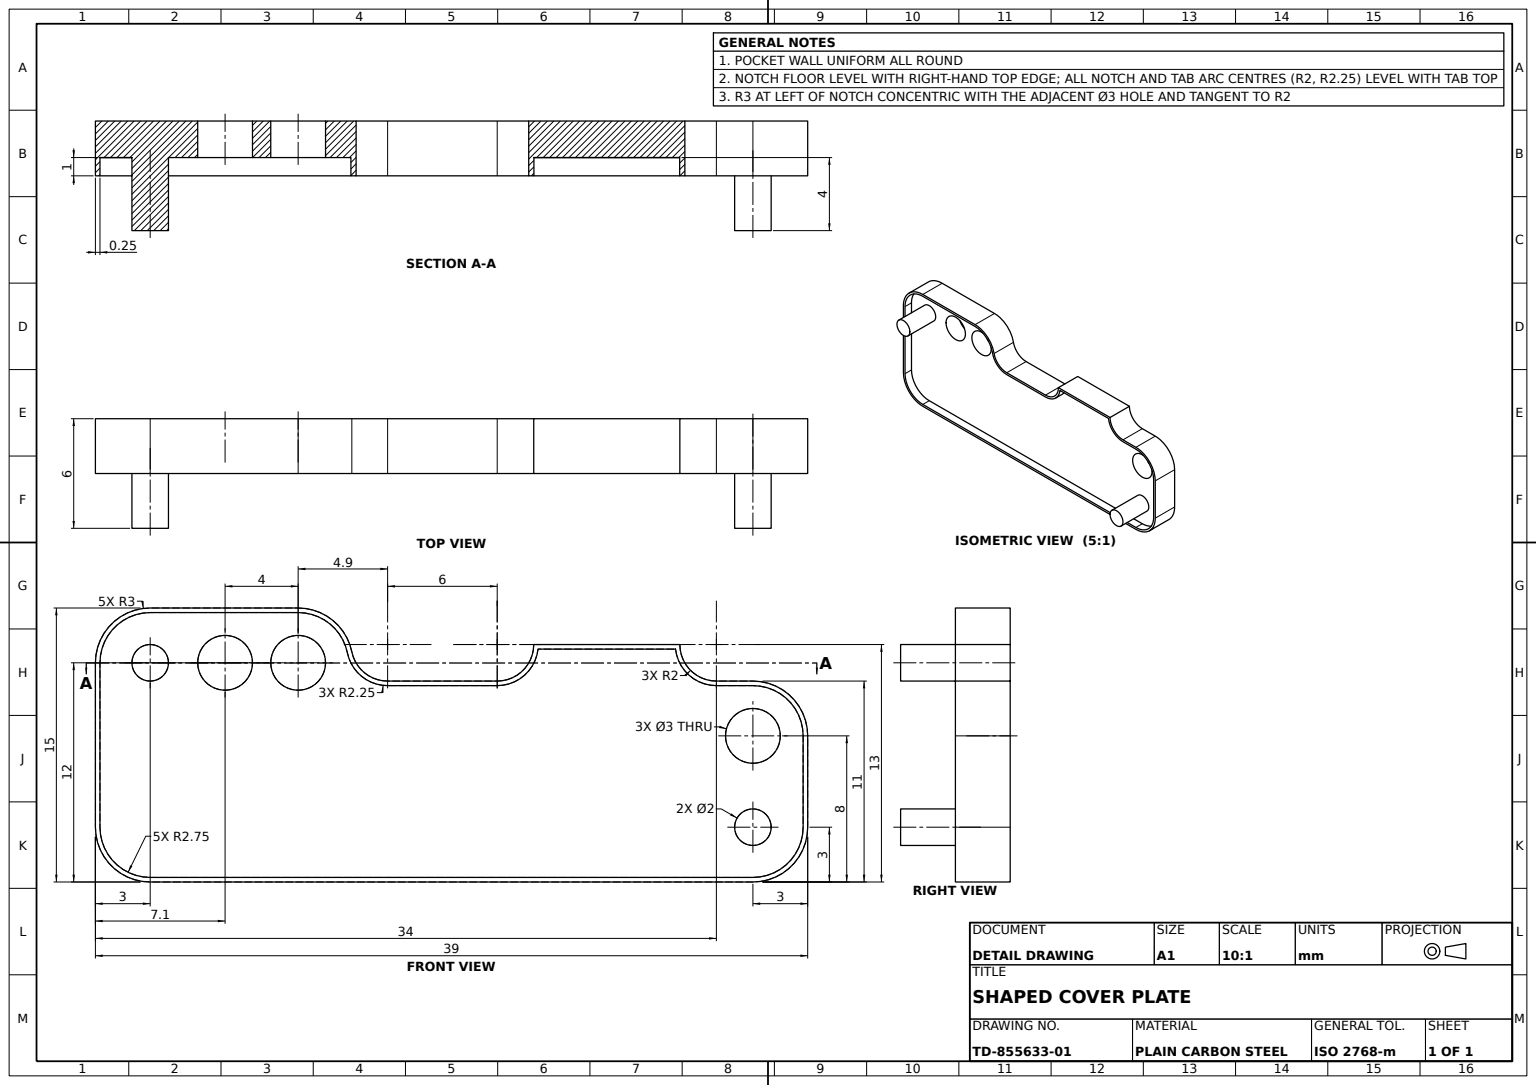
ISO-10303-21;
HEADER;
FILE_DESCRIPTION((''),'2;1');
FILE_NAME('','',(''),(''),'','','');
FILE_SCHEMA(('AUTOMOTIVE_DESIGN'));
ENDSEC;
DATA;
#1=APPLICATION_CONTEXT('');
#2=PRODUCT_CONTEXT('',#1,'mechanical');
#3=PRODUCT('','','',(#2));
#4=PRODUCT_DEFINITION_FORMATION('','',#3);
#5=PRODUCT_DEFINITION_CONTEXT('',#1,'design');
#6=PRODUCT_DEFINITION('','',#4,#5);
#7=PRODUCT_DEFINITION_SHAPE('','',#6);
#8=(LENGTH_UNIT()NAMED_UNIT(*)SI_UNIT(.MILLI.,.METRE.));
#9=(NAMED_UNIT(*)PLANE_ANGLE_UNIT()SI_UNIT($,.RADIAN.));
#10=(NAMED_UNIT(*)SI_UNIT($,.STERADIAN.)SOLID_ANGLE_UNIT());
#11=UNCERTAINTY_MEASURE_WITH_UNIT(LENGTH_MEASURE(1.E-05),#8,'distance_accuracy_value','');
#12=(GEOMETRIC_REPRESENTATION_CONTEXT(3)GLOBAL_UNCERTAINTY_ASSIGNED_CONTEXT((#11))GLOBAL_UNIT_ASSIGNED_CONTEXT((#8,#9,#10))REPRESENTATION_CONTEXT('',''));
#13=CARTESIAN_POINT('',(16.,10.75,2.));
#14=VERTEX_POINT('',#13);
#15=CARTESIAN_POINT('',(13.795459,12.55,2.));
#16=VERTEX_POINT('',#15);
#17=CARTESIAN_POINT('',(16.,13.,2.));
#18=DIRECTION('',(0.,0.,-1.));
#19=DIRECTION('',(1.,0.,0.));
#20=AXIS2_PLACEMENT_3D('',#17,#18,#19);
#21=CIRCLE('',#20,2.25);
#22=EDGE_CURVE('',#14,#16,#21,.T.);
#23=ORIENTED_EDGE('',*,*,#22,.F.);
#24=CARTESIAN_POINT('',(16.,10.75,3.));
#25=VERTEX_POINT('',#24);
#26=VECTOR('',#18,1000.);
#27=LINE('',#24,#26);
#28=EDGE_CURVE('',#25,#14,#27,.T.);
#29=ORIENTED_EDGE('',*,*,#28,.F.);
#30=CARTESIAN_POINT('',(13.795459,12.55,3.));
#31=VERTEX_POINT('',#30);
#32=CARTESIAN_POINT('',(16.,13.,3.));
#33=AXIS2_PLACEMENT_3D('',#32,#18,#19);
#34=CIRCLE('',#33,2.25);
#35=EDGE_CURVE('',#25,#31,#34,.T.);
#36=ORIENTED_EDGE('',*,*,#35,.T.);
#37=LINE('',#30,#26);
#38=EDGE_CURVE('',#31,#16,#37,.T.);
#39=ORIENTED_EDGE('',*,*,#38,.T.);
#40=EDGE_LOOP('',(#23,#29,#36,#39));
#41=FACE_OUTER_BOUND('',#40,.T.);
#42=DIRECTION('',(-1.,0.,0.));
#43=AXIS2_PLACEMENT_3D('',#32,#18,#42);
#44=CYLINDRICAL_SURFACE('',#43,2.25);
#45=ADVANCED_FACE('',(#41),#44,.T.);
#46=CARTESIAN_POINT('',(3.,15.,3.));
#47=VERTEX_POINT('',#46);
#48=CARTESIAN_POINT('',(3.,15.,0.));
#49=VERTEX_POINT('',#48);
#50=CARTESIAN_POINT('',(3.,15.,2.));
#51=LINE('',#50,#26);
#52=EDGE_CURVE('',#47,#49,#51,.T.);
#53=ORIENTED_EDGE('',*,*,#52,.F.);
#54=CARTESIAN_POINT('',(11.101021,15.,3.));
#55=VERTEX_POINT('',#54);
#56=VECTOR('',#42,1000.);
#57=LINE('',#54,#56);
#58=EDGE_CURVE('',#55,#47,#57,.T.);
#59=ORIENTED_EDGE('',*,*,#58,.F.);
#60=CARTESIAN_POINT('',(11.101021,15.,0.));
#61=VERTEX_POINT('',#60);
#62=CARTESIAN_POINT('',(11.101021,15.,2.));
#63=LINE('',#62,#26);
#64=EDGE_CURVE('',#55,#61,#63,.T.);
#65=ORIENTED_EDGE('',*,*,#64,.T.);
#66=LINE('',#60,#56);
#67=EDGE_CURVE('',#61,#49,#66,.T.);
#68=ORIENTED_EDGE('',*,*,#67,.T.);
#69=EDGE_LOOP('',(#53,#59,#65,#68));
#70=FACE_OUTER_BOUND('',#69,.T.);
#71=DIRECTION('',(0.,-1.,0.));
#72=AXIS2_PLACEMENT_3D('',#62,#71,#18);
#73=PLANE('',#72);
#74=ADVANCED_FACE('',(#70),#73,.F.);
#75=CARTESIAN_POINT('',(34.5,8.,0.));
#76=VERTEX_POINT('',#75);
#77=CARTESIAN_POINT('',(37.5,8.,0.));
#78=VERTEX_POINT('',#77);
#79=CARTESIAN_POINT('',(36.,8.,0.));
#80=DIRECTION('',(0.,0.,1.));
#81=AXIS2_PLACEMENT_3D('',#79,#80,#19);
#82=CIRCLE('',#81,1.5);
#83=EDGE_CURVE('',#76,#78,#82,.T.);
#84=ORIENTED_EDGE('',*,*,#83,.F.);
#85=CARTESIAN_POINT('',(34.5,8.,2.));
#86=VERTEX_POINT('',#85);
#87=CARTESIAN_POINT('',(34.5,8.,-2.));
#88=VECTOR('',#80,1000.);
#89=LINE('',#87,#88);
#90=EDGE_CURVE('',#76,#86,#89,.T.);
#91=ORIENTED_EDGE('',*,*,#90,.T.);
#92=CARTESIAN_POINT('',(37.5,8.,2.));
#93=VERTEX_POINT('',#92);
#94=CARTESIAN_POINT('',(36.,8.,2.));
#95=AXIS2_PLACEMENT_3D('',#94,#80,#19);
#96=CIRCLE('',#95,1.5);
#97=EDGE_CURVE('',#86,#93,#96,.T.);
#98=ORIENTED_EDGE('',*,*,#97,.T.);
#99=CARTESIAN_POINT('',(37.5,8.,-2.));
#100=LINE('',#99,#88);
#101=EDGE_CURVE('',#78,#93,#100,.T.);
#102=ORIENTED_EDGE('',*,*,#101,.F.);
#103=EDGE_LOOP('',(#84,#91,#98,#102));
#104=FACE_OUTER_BOUND('',#103,.T.);
#105=CARTESIAN_POINT('',(36.,8.,-2.));
#106=AXIS2_PLACEMENT_3D('',#105,#80,#19);
#107=CYLINDRICAL_SURFACE('',#106,1.5);
#108=ADVANCED_FACE('',(#104),#107,.F.);
#109=CARTESIAN_POINT('',(12.601021,12.,0.));
#110=VERTEX_POINT('',#109);
#111=CARTESIAN_POINT('',(9.601021,12.,0.));
#112=VERTEX_POINT('',#111);
#113=CARTESIAN_POINT('',(11.101021,12.,0.));
#114=AXIS2_PLACEMENT_3D('',#113,#80,#19);
#115=CIRCLE('',#114,1.5);
#116=EDGE_CURVE('',#110,#112,#115,.T.);
#117=ORIENTED_EDGE('',*,*,#116,.T.);
#118=EDGE_CURVE('',#112,#110,#115,.T.);
#119=ORIENTED_EDGE('',*,*,#118,.T.);
#120=EDGE_LOOP('',(#117,#119));
#121=FACE_BOUND('',#120,.T.);
#122=ORIENTED_EDGE('',*,*,#83,.T.);
#123=EDGE_CURVE('',#78,#76,#82,.T.);
#124=ORIENTED_EDGE('',*,*,#123,.T.);
#125=EDGE_LOOP('',(#122,#124));
#126=FACE_BOUND('',#125,.T.);
#127=CARTESIAN_POINT('',(5.601021,12.,0.));
#128=VERTEX_POINT('',#127);
#129=CARTESIAN_POINT('',(8.601021,12.,0.));
#130=VERTEX_POINT('',#129);
#131=CARTESIAN_POINT('',(7.101021,12.,0.));
#132=AXIS2_PLACEMENT_3D('',#131,#80,#19);
#133=CIRCLE('',#132,1.5);
#134=EDGE_CURVE('',#128,#130,#133,.T.);
#135=ORIENTED_EDGE('',*,*,#134,.T.);
#136=EDGE_CURVE('',#130,#128,#133,.T.);
#137=ORIENTED_EDGE('',*,*,#136,.T.);
#138=EDGE_LOOP('',(#135,#137));
#139=FACE_BOUND('',#138,.T.);
#140=CARTESIAN_POINT('',(0.,12.,0.));
#141=VERTEX_POINT('',#140);
#142=CARTESIAN_POINT('',(0.,3.,0.));
#143=VERTEX_POINT('',#142);
#144=VECTOR('',#71,1000.);
#145=LINE('',#142,#144);
#146=EDGE_CURVE('',#141,#143,#145,.T.);
#147=ORIENTED_EDGE('',*,*,#146,.F.);
#148=CARTESIAN_POINT('',(3.,12.,0.));
#149=AXIS2_PLACEMENT_3D('',#148,#80,#42);
#150=CIRCLE('',#149,3.);
#151=EDGE_CURVE('',#49,#141,#150,.T.);
#152=ORIENTED_EDGE('',*,*,#151,.F.);
#153=ORIENTED_EDGE('',*,*,#67,.F.);
#154=CARTESIAN_POINT('',(14.040408,12.6,0.));
#155=VERTEX_POINT('',#154);
#156=CIRCLE('',#114,3.);
#157=EDGE_CURVE('',#155,#61,#156,.T.);
#158=ORIENTED_EDGE('',*,*,#157,.F.);
#159=CARTESIAN_POINT('',(16.,11.,0.));
#160=VERTEX_POINT('',#159);
#161=CARTESIAN_POINT('',(16.,13.,0.));
#162=AXIS2_PLACEMENT_3D('',#161,#18,#42);
#163=CIRCLE('',#162,2.);
#164=EDGE_CURVE('',#160,#155,#163,.T.);
#165=ORIENTED_EDGE('',*,*,#164,.F.);
#166=CARTESIAN_POINT('',(22.,11.,0.));
#167=VERTEX_POINT('',#166);
#168=LINE('',#166,#56);
#169=EDGE_CURVE('',#167,#160,#168,.T.);
#170=ORIENTED_EDGE('',*,*,#169,.F.);
#171=CARTESIAN_POINT('',(24.,13.,0.));
#172=VERTEX_POINT('',#171);
#173=CARTESIAN_POINT('',(22.,13.,0.));
#174=AXIS2_PLACEMENT_3D('',#173,#18,#19);
#175=CIRCLE('',#174,2.);
#176=EDGE_CURVE('',#172,#167,#175,.T.);
#177=ORIENTED_EDGE('',*,*,#176,.F.);
#178=CARTESIAN_POINT('',(32.,13.,0.));
#179=VERTEX_POINT('',#178);
#180=LINE('',#178,#56);
#181=EDGE_CURVE('',#179,#172,#180,.T.);
#182=ORIENTED_EDGE('',*,*,#181,.F.);
#183=CARTESIAN_POINT('',(34.,11.,0.));
#184=VERTEX_POINT('',#183);
#185=CARTESIAN_POINT('',(34.,13.,0.));
#186=AXIS2_PLACEMENT_3D('',#185,#18,#19);
#187=CIRCLE('',#186,2.);
#188=EDGE_CURVE('',#184,#179,#187,.T.);
#189=ORIENTED_EDGE('',*,*,#188,.F.);
#190=CARTESIAN_POINT('',(36.,11.,0.));
#191=VERTEX_POINT('',#190);
#192=LINE('',#190,#56);
#193=EDGE_CURVE('',#191,#184,#192,.T.);
#194=ORIENTED_EDGE('',*,*,#193,.F.);
#195=CARTESIAN_POINT('',(39.,8.,0.));
#196=VERTEX_POINT('',#195);
#197=CIRCLE('',#81,3.);
#198=EDGE_CURVE('',#196,#191,#197,.T.);
#199=ORIENTED_EDGE('',*,*,#198,.F.);
#200=CARTESIAN_POINT('',(39.,3.,0.));
#201=VERTEX_POINT('',#200);
#202=DIRECTION('',(0.,1.,0.));
#203=VECTOR('',#202,1000.);
#204=LINE('',#200,#203);
#205=EDGE_CURVE('',#201,#196,#204,.T.);
#206=ORIENTED_EDGE('',*,*,#205,.F.);
#207=CARTESIAN_POINT('',(36.,0.,0.));
#208=VERTEX_POINT('',#207);
#209=CARTESIAN_POINT('',(36.,3.,0.));
#210=AXIS2_PLACEMENT_3D('',#209,#80,#19);
#211=CIRCLE('',#210,3.);
#212=EDGE_CURVE('',#208,#201,#211,.T.);
#213=ORIENTED_EDGE('',*,*,#212,.F.);
#214=CARTESIAN_POINT('',(3.,0.,0.));
#215=VERTEX_POINT('',#214);
#216=VECTOR('',#19,1000.);
#217=LINE('',#214,#216);
#218=EDGE_CURVE('',#215,#208,#217,.T.);
#219=ORIENTED_EDGE('',*,*,#218,.F.);
#220=CARTESIAN_POINT('',(3.,3.,0.));
#221=AXIS2_PLACEMENT_3D('',#220,#80,#19);
#222=CIRCLE('',#221,3.);
#223=EDGE_CURVE('',#143,#215,#222,.T.);
#224=ORIENTED_EDGE('',*,*,#223,.F.);
#225=EDGE_LOOP('',(#147,#152,#153,#158,#165,#170,#177,#182,#189,#194,#199,#206,#213,#219,#224));
#226=FACE_OUTER_BOUND('',#225,.T.);
#227=AXIS2_PLACEMENT_3D('',#185,#80,#19);
#228=PLANE('',#227);
#229=ADVANCED_FACE('',(#121,#126,#139,#226),#228,.F.);
#230=CARTESIAN_POINT('',(3.,14.75,3.));
#231=VERTEX_POINT('',#230);
#232=CARTESIAN_POINT('',(0.25,12.,3.));
#233=VERTEX_POINT('',#232);
#234=CARTESIAN_POINT('',(3.,12.,3.));
#235=AXIS2_PLACEMENT_3D('',#234,#80,#19);
#236=CIRCLE('',#235,2.75);
#237=EDGE_CURVE('',#231,#233,#236,.T.);
#238=ORIENTED_EDGE('',*,*,#237,.T.);
#239=CARTESIAN_POINT('',(0.25,12.,2.));
#240=VERTEX_POINT('',#239);
#241=LINE('',#232,#26);
#242=EDGE_CURVE('',#233,#240,#241,.T.);
#243=ORIENTED_EDGE('',*,*,#242,.T.);
#244=CARTESIAN_POINT('',(3.,14.75,2.));
#245=VERTEX_POINT('',#244);
#246=CARTESIAN_POINT('',(3.,12.,2.));
#247=AXIS2_PLACEMENT_3D('',#246,#80,#19);
#248=CIRCLE('',#247,2.75);
#249=EDGE_CURVE('',#245,#240,#248,.T.);
#250=ORIENTED_EDGE('',*,*,#249,.F.);
#251=LINE('',#230,#26);
#252=EDGE_CURVE('',#231,#245,#251,.T.);
#253=ORIENTED_EDGE('',*,*,#252,.F.);
#254=EDGE_LOOP('',(#238,#243,#250,#253));
#255=FACE_OUTER_BOUND('',#254,.T.);
#256=AXIS2_PLACEMENT_3D('',#234,#18,#42);
#257=CYLINDRICAL_SURFACE('',#256,2.75);
#258=ADVANCED_FACE('',(#255),#257,.F.);
#259=CARTESIAN_POINT('',(0.25,3.,3.));
#260=VERTEX_POINT('',#259);
#261=CARTESIAN_POINT('',(0.25,3.,2.));
#262=VERTEX_POINT('',#261);
#263=LINE('',#259,#26);
#264=EDGE_CURVE('',#260,#262,#263,.T.);
#265=ORIENTED_EDGE('',*,*,#264,.F.);
#266=CARTESIAN_POINT('',(3.,0.25,3.));
#267=VERTEX_POINT('',#266);
#268=CARTESIAN_POINT('',(3.,3.,3.));
#269=AXIS2_PLACEMENT_3D('',#268,#80,#19);
#270=CIRCLE('',#269,2.75);
#271=EDGE_CURVE('',#260,#267,#270,.T.);
#272=ORIENTED_EDGE('',*,*,#271,.T.);
#273=CARTESIAN_POINT('',(3.,0.25,2.));
#274=VERTEX_POINT('',#273);
#275=LINE('',#266,#26);
#276=EDGE_CURVE('',#267,#274,#275,.T.);
#277=ORIENTED_EDGE('',*,*,#276,.T.);
#278=CARTESIAN_POINT('',(3.,3.,2.));
#279=AXIS2_PLACEMENT_3D('',#278,#80,#19);
#280=CIRCLE('',#279,2.75);
#281=EDGE_CURVE('',#262,#274,#280,.T.);
#282=ORIENTED_EDGE('',*,*,#281,.F.);
#283=EDGE_LOOP('',(#265,#272,#277,#282));
#284=FACE_OUTER_BOUND('',#283,.T.);
#285=AXIS2_PLACEMENT_3D('',#268,#18,#42);
#286=CYLINDRICAL_SURFACE('',#285,2.75);
#287=ADVANCED_FACE('',(#284),#286,.F.);
#288=ORIENTED_EDGE('',*,*,#58,.T.);
#289=CARTESIAN_POINT('',(0.,12.,3.));
#290=VERTEX_POINT('',#289);
#291=CIRCLE('',#235,3.);
#292=EDGE_CURVE('',#47,#290,#291,.T.);
#293=ORIENTED_EDGE('',*,*,#292,.T.);
#294=CARTESIAN_POINT('',(0.,3.,3.));
#295=VERTEX_POINT('',#294);
#296=LINE('',#289,#144);
#297=EDGE_CURVE('',#290,#295,#296,.T.);
#298=ORIENTED_EDGE('',*,*,#297,.T.);
#299=CARTESIAN_POINT('',(3.,0.,3.));
#300=VERTEX_POINT('',#299);
#301=CIRCLE('',#269,3.);
#302=EDGE_CURVE('',#295,#300,#301,.T.);
#303=ORIENTED_EDGE('',*,*,#302,.T.);
#304=CARTESIAN_POINT('',(36.,0.,3.));
#305=VERTEX_POINT('',#304);
#306=LINE('',#299,#216);
#307=EDGE_CURVE('',#300,#305,#306,.T.);
#308=ORIENTED_EDGE('',*,*,#307,.T.);
#309=CARTESIAN_POINT('',(39.,3.,3.));
#310=VERTEX_POINT('',#309);
#311=CARTESIAN_POINT('',(36.,3.,3.));
#312=AXIS2_PLACEMENT_3D('',#311,#80,#19);
#313=CIRCLE('',#312,3.);
#314=EDGE_CURVE('',#305,#310,#313,.T.);
#315=ORIENTED_EDGE('',*,*,#314,.T.);
#316=CARTESIAN_POINT('',(39.,8.,3.));
#317=VERTEX_POINT('',#316);
#318=LINE('',#309,#203);
#319=EDGE_CURVE('',#310,#317,#318,.T.);
#320=ORIENTED_EDGE('',*,*,#319,.T.);
#321=CARTESIAN_POINT('',(36.,11.,3.));
#322=VERTEX_POINT('',#321);
#323=CARTESIAN_POINT('',(36.,8.,3.));
#324=AXIS2_PLACEMENT_3D('',#323,#80,#19);
#325=CIRCLE('',#324,3.);
#326=EDGE_CURVE('',#317,#322,#325,.T.);
#327=ORIENTED_EDGE('',*,*,#326,.T.);
#328=CARTESIAN_POINT('',(34.,11.,3.));
#329=VERTEX_POINT('',#328);
#330=LINE('',#321,#56);
#331=EDGE_CURVE('',#322,#329,#330,.T.);
#332=ORIENTED_EDGE('',*,*,#331,.T.);
#333=CARTESIAN_POINT('',(32.,13.,3.));
#334=VERTEX_POINT('',#333);
#335=CARTESIAN_POINT('',(34.,13.,3.));
#336=AXIS2_PLACEMENT_3D('',#335,#18,#19);
#337=CIRCLE('',#336,2.);
#338=EDGE_CURVE('',#329,#334,#337,.T.);
#339=ORIENTED_EDGE('',*,*,#338,.T.);
#340=CARTESIAN_POINT('',(24.,13.,3.));
#341=VERTEX_POINT('',#340);
#342=LINE('',#333,#56);
#343=EDGE_CURVE('',#334,#341,#342,.T.);
#344=ORIENTED_EDGE('',*,*,#343,.T.);
#345=CARTESIAN_POINT('',(22.,11.,3.));
#346=VERTEX_POINT('',#345);
#347=CARTESIAN_POINT('',(22.,13.,3.));
#348=AXIS2_PLACEMENT_3D('',#347,#18,#19);
#349=CIRCLE('',#348,2.);
#350=EDGE_CURVE('',#341,#346,#349,.T.);
#351=ORIENTED_EDGE('',*,*,#350,.T.);
#352=CARTESIAN_POINT('',(16.,11.,3.));
#353=VERTEX_POINT('',#352);
#354=LINE('',#345,#56);
#355=EDGE_CURVE('',#346,#353,#354,.T.);
#356=ORIENTED_EDGE('',*,*,#355,.T.);
#357=CARTESIAN_POINT('',(14.040408,12.6,3.));
#358=VERTEX_POINT('',#357);
#359=CIRCLE('',#33,2.);
#360=EDGE_CURVE('',#353,#358,#359,.T.);
#361=ORIENTED_EDGE('',*,*,#360,.T.);
#362=CARTESIAN_POINT('',(11.101021,12.,3.));
#363=AXIS2_PLACEMENT_3D('',#362,#80,#19);
#364=CIRCLE('',#363,3.);
#365=EDGE_CURVE('',#358,#55,#364,.T.);
#366=ORIENTED_EDGE('',*,*,#365,.T.);
#367=EDGE_LOOP('',(#288,#293,#298,#303,#308,#315,#320,#327,#332,#339,#344,#351,#356,#361,#366));
#368=FACE_OUTER_BOUND('',#367,.T.);
#369=CARTESIAN_POINT('',(38.75,8.,3.));
#370=VERTEX_POINT('',#369);
#371=CARTESIAN_POINT('',(36.,10.75,3.));
#372=VERTEX_POINT('',#371);
#373=CIRCLE('',#324,2.75);
#374=EDGE_CURVE('',#370,#372,#373,.T.);
#375=ORIENTED_EDGE('',*,*,#374,.F.);
#376=CARTESIAN_POINT('',(38.75,3.,3.));
#377=VERTEX_POINT('',#376);
#378=LINE('',#376,#203);
#379=EDGE_CURVE('',#377,#370,#378,.T.);
#380=ORIENTED_EDGE('',*,*,#379,.F.);
#381=CARTESIAN_POINT('',(36.,0.25,3.));
#382=VERTEX_POINT('',#381);
#383=CIRCLE('',#312,2.75);
#384=EDGE_CURVE('',#382,#377,#383,.T.);
#385=ORIENTED_EDGE('',*,*,#384,.F.);
#386=LINE('',#266,#216);
#387=EDGE_CURVE('',#267,#382,#386,.T.);
#388=ORIENTED_EDGE('',*,*,#387,.F.);
#389=ORIENTED_EDGE('',*,*,#271,.F.);
#390=LINE('',#232,#144);
#391=EDGE_CURVE('',#233,#260,#390,.T.);
#392=ORIENTED_EDGE('',*,*,#391,.F.);
#393=ORIENTED_EDGE('',*,*,#237,.F.);
#394=CARTESIAN_POINT('',(11.101021,14.75,3.));
#395=VERTEX_POINT('',#394);
#396=LINE('',#394,#56);
#397=EDGE_CURVE('',#395,#231,#396,.T.);
#398=ORIENTED_EDGE('',*,*,#397,.F.);
#399=CIRCLE('',#363,2.75);
#400=EDGE_CURVE('',#31,#395,#399,.T.);
#401=ORIENTED_EDGE('',*,*,#400,.F.);
#402=ORIENTED_EDGE('',*,*,#35,.F.);
#403=CARTESIAN_POINT('',(22.,10.75,3.));
#404=VERTEX_POINT('',#403);
#405=LINE('',#403,#56);
#406=EDGE_CURVE('',#404,#25,#405,.T.);
#407=ORIENTED_EDGE('',*,*,#406,.F.);
#408=CARTESIAN_POINT('',(24.236068,12.75,3.));
#409=VERTEX_POINT('',#408);
#410=CIRCLE('',#348,2.25);
#411=EDGE_CURVE('',#409,#404,#410,.T.);
#412=ORIENTED_EDGE('',*,*,#411,.F.);
#413=CARTESIAN_POINT('',(31.763932,12.75,3.));
#414=VERTEX_POINT('',#413);
#415=LINE('',#413,#56);
#416=EDGE_CURVE('',#414,#409,#415,.T.);
#417=ORIENTED_EDGE('',*,*,#416,.F.);
#418=CARTESIAN_POINT('',(34.,10.75,3.));
#419=VERTEX_POINT('',#418);
#420=CIRCLE('',#336,2.25);
#421=EDGE_CURVE('',#419,#414,#420,.T.);
#422=ORIENTED_EDGE('',*,*,#421,.F.);
#423=LINE('',#371,#56);
#424=EDGE_CURVE('',#372,#419,#423,.T.);
#425=ORIENTED_EDGE('',*,*,#424,.F.);
#426=EDGE_LOOP('',(#375,#380,#385,#388,#389,#392,#393,#398,#401,#402,#407,#412,#417,#422,#425));
#427=FACE_BOUND('',#426,.T.);
#428=AXIS2_PLACEMENT_3D('',#335,#80,#19);
#429=PLANE('',#428);
#430=ADVANCED_FACE('',(#368,#427),#429,.T.);
#431=ORIENTED_EDGE('',*,*,#400,.T.);
#432=CARTESIAN_POINT('',(11.101021,14.75,2.));
#433=VERTEX_POINT('',#432);
#434=LINE('',#394,#26);
#435=EDGE_CURVE('',#395,#433,#434,.T.);
#436=ORIENTED_EDGE('',*,*,#435,.T.);
#437=CARTESIAN_POINT('',(11.101021,12.,2.));
#438=AXIS2_PLACEMENT_3D('',#437,#80,#19);
#439=CIRCLE('',#438,2.75);
#440=EDGE_CURVE('',#16,#433,#439,.T.);
#441=ORIENTED_EDGE('',*,*,#440,.F.);
#442=ORIENTED_EDGE('',*,*,#38,.F.);
#443=EDGE_LOOP('',(#431,#436,#441,#442));
#444=FACE_OUTER_BOUND('',#443,.T.);
#445=AXIS2_PLACEMENT_3D('',#362,#18,#42);
#446=CYLINDRICAL_SURFACE('',#445,2.75);
#447=ADVANCED_FACE('',(#444),#446,.F.);
#448=CARTESIAN_POINT('',(34.,10.75,2.));
#449=VERTEX_POINT('',#448);
#450=LINE('',#418,#26);
#451=EDGE_CURVE('',#419,#449,#450,.T.);
#452=ORIENTED_EDGE('',*,*,#451,.F.);
#453=ORIENTED_EDGE('',*,*,#421,.T.);
#454=CARTESIAN_POINT('',(31.763932,12.75,2.));
#455=VERTEX_POINT('',#454);
#456=LINE('',#413,#26);
#457=EDGE_CURVE('',#414,#455,#456,.T.);
#458=ORIENTED_EDGE('',*,*,#457,.T.);
#459=CARTESIAN_POINT('',(34.,13.,2.));
#460=AXIS2_PLACEMENT_3D('',#459,#18,#19);
#461=CIRCLE('',#460,2.25);
#462=EDGE_CURVE('',#449,#455,#461,.T.);
#463=ORIENTED_EDGE('',*,*,#462,.F.);
#464=EDGE_LOOP('',(#452,#453,#458,#463));
#465=FACE_OUTER_BOUND('',#464,.T.);
#466=AXIS2_PLACEMENT_3D('',#335,#18,#42);
#467=CYLINDRICAL_SURFACE('',#466,2.25);
#468=ADVANCED_FACE('',(#465),#467,.T.);
#469=CARTESIAN_POINT('',(12.601021,12.,2.));
#470=VERTEX_POINT('',#469);
#471=CARTESIAN_POINT('',(12.601021,12.,-2.));
#472=LINE('',#471,#88);
#473=EDGE_CURVE('',#110,#470,#472,.T.);
#474=ORIENTED_EDGE('',*,*,#473,.F.);
#475=ORIENTED_EDGE('',*,*,#118,.F.);
#476=CARTESIAN_POINT('',(9.601021,12.,2.));
#477=VERTEX_POINT('',#476);
#478=CARTESIAN_POINT('',(9.601021,12.,-2.));
#479=LINE('',#478,#88);
#480=EDGE_CURVE('',#112,#477,#479,.T.);
#481=ORIENTED_EDGE('',*,*,#480,.T.);
#482=CIRCLE('',#438,1.5);
#483=EDGE_CURVE('',#477,#470,#482,.T.);
#484=ORIENTED_EDGE('',*,*,#483,.T.);
#485=EDGE_LOOP('',(#474,#475,#481,#484));
#486=FACE_OUTER_BOUND('',#485,.T.);
#487=CARTESIAN_POINT('',(11.101021,12.,-2.));
#488=AXIS2_PLACEMENT_3D('',#487,#80,#19);
#489=CYLINDRICAL_SURFACE('',#488,1.5);
#490=ADVANCED_FACE('',(#486),#489,.F.);
#491=CARTESIAN_POINT('',(16.,11.,2.));
#492=LINE('',#491,#26);
#493=EDGE_CURVE('',#353,#160,#492,.T.);
#494=ORIENTED_EDGE('',*,*,#493,.T.);
#495=ORIENTED_EDGE('',*,*,#164,.T.);
#496=CARTESIAN_POINT('',(14.040408,12.6,2.));
#497=LINE('',#496,#26);
#498=EDGE_CURVE('',#358,#155,#497,.T.);
#499=ORIENTED_EDGE('',*,*,#498,.F.);
#500=ORIENTED_EDGE('',*,*,#360,.F.);
#501=EDGE_LOOP('',(#494,#495,#499,#500));
#502=FACE_OUTER_BOUND('',#501,.T.);
#503=AXIS2_PLACEMENT_3D('',#17,#18,#42);
#504=CYLINDRICAL_SURFACE('',#503,2.);
#505=ADVANCED_FACE('',(#502),#504,.F.);
#506=ORIENTED_EDGE('',*,*,#374,.T.);
#507=CARTESIAN_POINT('',(36.,10.75,2.));
#508=VERTEX_POINT('',#507);
#509=LINE('',#371,#26);
#510=EDGE_CURVE('',#372,#508,#509,.T.);
#511=ORIENTED_EDGE('',*,*,#510,.T.);
#512=CARTESIAN_POINT('',(38.75,8.,2.));
#513=VERTEX_POINT('',#512);
#514=CIRCLE('',#95,2.75);
#515=EDGE_CURVE('',#513,#508,#514,.T.);
#516=ORIENTED_EDGE('',*,*,#515,.F.);
#517=LINE('',#369,#26);
#518=EDGE_CURVE('',#370,#513,#517,.T.);
#519=ORIENTED_EDGE('',*,*,#518,.F.);
#520=EDGE_LOOP('',(#506,#511,#516,#519));
#521=FACE_OUTER_BOUND('',#520,.T.);
#522=AXIS2_PLACEMENT_3D('',#323,#18,#42);
#523=CYLINDRICAL_SURFACE('',#522,2.75);
#524=ADVANCED_FACE('',(#521),#523,.F.);
#525=ORIENTED_EDGE('',*,*,#146,.T.);
#526=CARTESIAN_POINT('',(0.,3.,2.));
#527=LINE('',#526,#26);
#528=EDGE_CURVE('',#295,#143,#527,.T.);
#529=ORIENTED_EDGE('',*,*,#528,.F.);
#530=ORIENTED_EDGE('',*,*,#297,.F.);
#531=CARTESIAN_POINT('',(0.,12.,2.));
#532=LINE('',#531,#26);
#533=EDGE_CURVE('',#290,#141,#532,.T.);
#534=ORIENTED_EDGE('',*,*,#533,.T.);
#535=EDGE_LOOP('',(#525,#529,#530,#534));
#536=FACE_OUTER_BOUND('',#535,.T.);
#537=AXIS2_PLACEMENT_3D('',#526,#19,#18);
#538=PLANE('',#537);
#539=ADVANCED_FACE('',(#536),#538,.F.);
#540=LINE('',#507,#56);
#541=EDGE_CURVE('',#508,#449,#540,.T.);
#542=ORIENTED_EDGE('',*,*,#541,.F.);
#543=ORIENTED_EDGE('',*,*,#510,.F.);
#544=ORIENTED_EDGE('',*,*,#424,.T.);
#545=ORIENTED_EDGE('',*,*,#451,.T.);
#546=EDGE_LOOP('',(#542,#543,#544,#545));
#547=FACE_OUTER_BOUND('',#546,.T.);
#548=AXIS2_PLACEMENT_3D('',#371,#71,#19);
#549=PLANE('',#548);
#550=ADVANCED_FACE('',(#547),#549,.T.);
#551=LINE('',#239,#144);
#552=EDGE_CURVE('',#240,#262,#551,.T.);
#553=ORIENTED_EDGE('',*,*,#552,.F.);
#554=ORIENTED_EDGE('',*,*,#242,.F.);
#555=ORIENTED_EDGE('',*,*,#391,.T.);
#556=ORIENTED_EDGE('',*,*,#264,.T.);
#557=EDGE_LOOP('',(#553,#554,#555,#556));
#558=FACE_OUTER_BOUND('',#557,.T.);
#559=AXIS2_PLACEMENT_3D('',#232,#19,#202);
#560=PLANE('',#559);
#561=ADVANCED_FACE('',(#558),#560,.T.);
#562=CARTESIAN_POINT('',(2.,12.,6.));
#563=VERTEX_POINT('',#562);
#564=CARTESIAN_POINT('',(4.,12.,6.));
#565=VERTEX_POINT('',#564);
#566=CARTESIAN_POINT('',(3.,12.,6.));
#567=AXIS2_PLACEMENT_3D('',#566,#80,#19);
#568=CIRCLE('',#567,1.);
#569=EDGE_CURVE('',#563,#565,#568,.T.);
#570=ORIENTED_EDGE('',*,*,#569,.T.);
#571=EDGE_CURVE('',#565,#563,#568,.T.);
#572=ORIENTED_EDGE('',*,*,#571,.T.);
#573=EDGE_LOOP('',(#570,#572));
#574=FACE_OUTER_BOUND('',#573,.T.);
#575=PLANE('',#567);
#576=ADVANCED_FACE('',(#574),#575,.T.);
#577=CARTESIAN_POINT('',(36.,0.25,2.));
#578=VERTEX_POINT('',#577);
#579=LINE('',#381,#26);
#580=EDGE_CURVE('',#382,#578,#579,.T.);
#581=ORIENTED_EDGE('',*,*,#580,.T.);
#582=LINE('',#273,#216);
#583=EDGE_CURVE('',#274,#578,#582,.T.);
#584=ORIENTED_EDGE('',*,*,#583,.F.);
#585=ORIENTED_EDGE('',*,*,#276,.F.);
#586=ORIENTED_EDGE('',*,*,#387,.T.);
#587=EDGE_LOOP('',(#581,#584,#585,#586));
#588=FACE_OUTER_BOUND('',#587,.T.);
#589=AXIS2_PLACEMENT_3D('',#266,#202,#42);
#590=PLANE('',#589);
#591=ADVANCED_FACE('',(#588),#590,.T.);
#592=CARTESIAN_POINT('',(2.,12.,2.));
#593=VERTEX_POINT('',#592);
#594=LINE('',#562,#26);
#595=EDGE_CURVE('',#563,#593,#594,.T.);
#596=ORIENTED_EDGE('',*,*,#595,.F.);
#597=ORIENTED_EDGE('',*,*,#571,.F.);
#598=CARTESIAN_POINT('',(4.,12.,2.));
#599=VERTEX_POINT('',#598);
#600=LINE('',#564,#26);
#601=EDGE_CURVE('',#565,#599,#600,.T.);
#602=ORIENTED_EDGE('',*,*,#601,.T.);
#603=CIRCLE('',#247,1.);
#604=EDGE_CURVE('',#599,#593,#603,.T.);
#605=ORIENTED_EDGE('',*,*,#604,.T.);
#606=EDGE_LOOP('',(#596,#597,#602,#605));
#607=FACE_OUTER_BOUND('',#606,.T.);
#608=AXIS2_PLACEMENT_3D('',#566,#18,#42);
#609=CYLINDRICAL_SURFACE('',#608,1.);
#610=ADVANCED_FACE('',(#607),#609,.T.);
#611=ORIENTED_EDGE('',*,*,#480,.F.);
#612=ORIENTED_EDGE('',*,*,#116,.F.);
#613=ORIENTED_EDGE('',*,*,#473,.T.);
#614=EDGE_CURVE('',#470,#477,#482,.T.);
#615=ORIENTED_EDGE('',*,*,#614,.T.);
#616=EDGE_LOOP('',(#611,#612,#613,#615));
#617=FACE_OUTER_BOUND('',#616,.T.);
#618=ADVANCED_FACE('',(#617),#489,.F.);
#619=CARTESIAN_POINT('',(39.,3.,2.));
#620=LINE('',#619,#26);
#621=EDGE_CURVE('',#310,#201,#620,.T.);
#622=ORIENTED_EDGE('',*,*,#621,.T.);
#623=ORIENTED_EDGE('',*,*,#205,.T.);
#624=CARTESIAN_POINT('',(39.,8.,2.));
#625=LINE('',#624,#26);
#626=EDGE_CURVE('',#317,#196,#625,.T.);
#627=ORIENTED_EDGE('',*,*,#626,.F.);
#628=ORIENTED_EDGE('',*,*,#319,.F.);
#629=EDGE_LOOP('',(#622,#623,#627,#628));
#630=FACE_OUTER_BOUND('',#629,.T.);
#631=AXIS2_PLACEMENT_3D('',#619,#42,#80);
#632=PLANE('',#631);
#633=ADVANCED_FACE('',(#630),#632,.F.);
#634=ORIENTED_EDGE('',*,*,#498,.T.);
#635=ORIENTED_EDGE('',*,*,#157,.T.);
#636=ORIENTED_EDGE('',*,*,#64,.F.);
#637=ORIENTED_EDGE('',*,*,#365,.F.);
#638=EDGE_LOOP('',(#634,#635,#636,#637));
#639=FACE_OUTER_BOUND('',#638,.T.);
#640=AXIS2_PLACEMENT_3D('',#437,#18,#42);
#641=CYLINDRICAL_SURFACE('',#640,3.);
#642=ADVANCED_FACE('',(#639),#641,.T.);
#643=CARTESIAN_POINT('',(38.75,3.,2.));
#644=VERTEX_POINT('',#643);
#645=CARTESIAN_POINT('',(36.,3.,2.));
#646=AXIS2_PLACEMENT_3D('',#645,#80,#19);
#647=CIRCLE('',#646,2.75);
#648=EDGE_CURVE('',#578,#644,#647,.T.);
#649=ORIENTED_EDGE('',*,*,#648,.F.);
#650=ORIENTED_EDGE('',*,*,#580,.F.);
#651=ORIENTED_EDGE('',*,*,#384,.T.);
#652=LINE('',#376,#26);
#653=EDGE_CURVE('',#377,#644,#652,.T.);
#654=ORIENTED_EDGE('',*,*,#653,.T.);
#655=EDGE_LOOP('',(#649,#650,#651,#654));
#656=FACE_OUTER_BOUND('',#655,.T.);
#657=AXIS2_PLACEMENT_3D('',#311,#18,#42);
#658=CYLINDRICAL_SURFACE('',#657,2.75);
#659=ADVANCED_FACE('',(#656),#658,.F.);
#660=CARTESIAN_POINT('',(36.,11.,2.));
#661=LINE('',#660,#26);
#662=EDGE_CURVE('',#322,#191,#661,.T.);
#663=ORIENTED_EDGE('',*,*,#662,.F.);
#664=ORIENTED_EDGE('',*,*,#326,.F.);
#665=ORIENTED_EDGE('',*,*,#626,.T.);
#666=ORIENTED_EDGE('',*,*,#198,.T.);
#667=EDGE_LOOP('',(#663,#664,#665,#666));
#668=FACE_OUTER_BOUND('',#667,.T.);
#669=AXIS2_PLACEMENT_3D('',#94,#18,#42);
#670=CYLINDRICAL_SURFACE('',#669,3.);
#671=ADVANCED_FACE('',(#668),#670,.T.);
#672=ORIENTED_EDGE('',*,*,#662,.T.);
#673=ORIENTED_EDGE('',*,*,#193,.T.);
#674=CARTESIAN_POINT('',(34.,11.,2.));
#675=LINE('',#674,#26);
#676=EDGE_CURVE('',#329,#184,#675,.T.);
#677=ORIENTED_EDGE('',*,*,#676,.F.);
#678=ORIENTED_EDGE('',*,*,#331,.F.);
#679=EDGE_LOOP('',(#672,#673,#677,#678));
#680=FACE_OUTER_BOUND('',#679,.T.);
#681=AXIS2_PLACEMENT_3D('',#660,#71,#18);
#682=PLANE('',#681);
#683=ADVANCED_FACE('',(#680),#682,.F.);
#684=CARTESIAN_POINT('',(35.,3.,2.));
#685=VERTEX_POINT('',#684);
#686=CARTESIAN_POINT('',(37.,3.,2.));
#687=VERTEX_POINT('',#686);
#688=CIRCLE('',#646,1.);
#689=EDGE_CURVE('',#685,#687,#688,.T.);
#690=ORIENTED_EDGE('',*,*,#689,.T.);
#691=CARTESIAN_POINT('',(37.,3.,6.));
#692=VERTEX_POINT('',#691);
#693=LINE('',#691,#26);
#694=EDGE_CURVE('',#692,#687,#693,.T.);
#695=ORIENTED_EDGE('',*,*,#694,.F.);
#696=CARTESIAN_POINT('',(35.,3.,6.));
#697=VERTEX_POINT('',#696);
#698=CARTESIAN_POINT('',(36.,3.,6.));
#699=AXIS2_PLACEMENT_3D('',#698,#80,#19);
#700=CIRCLE('',#699,1.);
#701=EDGE_CURVE('',#697,#692,#700,.T.);
#702=ORIENTED_EDGE('',*,*,#701,.F.);
#703=LINE('',#696,#26);
#704=EDGE_CURVE('',#697,#685,#703,.T.);
#705=ORIENTED_EDGE('',*,*,#704,.T.);
#706=EDGE_LOOP('',(#690,#695,#702,#705));
#707=FACE_OUTER_BOUND('',#706,.T.);
#708=AXIS2_PLACEMENT_3D('',#698,#18,#42);
#709=CYLINDRICAL_SURFACE('',#708,1.);
#710=ADVANCED_FACE('',(#707),#709,.T.);
#711=EDGE_CURVE('',#93,#86,#96,.T.);
#712=ORIENTED_EDGE('',*,*,#711,.T.);
#713=ORIENTED_EDGE('',*,*,#90,.F.);
#714=ORIENTED_EDGE('',*,*,#123,.F.);
#715=ORIENTED_EDGE('',*,*,#101,.T.);
#716=EDGE_LOOP('',(#712,#713,#714,#715));
#717=FACE_OUTER_BOUND('',#716,.T.);
#718=ADVANCED_FACE('',(#717),#107,.F.);
#719=ORIENTED_EDGE('',*,*,#411,.T.);
#720=CARTESIAN_POINT('',(22.,10.75,2.));
#721=VERTEX_POINT('',#720);
#722=LINE('',#403,#26);
#723=EDGE_CURVE('',#404,#721,#722,.T.);
#724=ORIENTED_EDGE('',*,*,#723,.T.);
#725=CARTESIAN_POINT('',(24.236068,12.75,2.));
#726=VERTEX_POINT('',#725);
#727=CARTESIAN_POINT('',(22.,13.,2.));
#728=AXIS2_PLACEMENT_3D('',#727,#18,#19);
#729=CIRCLE('',#728,2.25);
#730=EDGE_CURVE('',#726,#721,#729,.T.);
#731=ORIENTED_EDGE('',*,*,#730,.F.);
#732=LINE('',#408,#26);
#733=EDGE_CURVE('',#409,#726,#732,.T.);
#734=ORIENTED_EDGE('',*,*,#733,.F.);
#735=EDGE_LOOP('',(#719,#724,#731,#734));
#736=FACE_OUTER_BOUND('',#735,.T.);
#737=AXIS2_PLACEMENT_3D('',#347,#18,#42);
#738=CYLINDRICAL_SURFACE('',#737,2.25);
#739=ADVANCED_FACE('',(#736),#738,.T.);
#740=CARTESIAN_POINT('',(24.,13.,2.));
#741=LINE('',#740,#26);
#742=EDGE_CURVE('',#341,#172,#741,.T.);
#743=ORIENTED_EDGE('',*,*,#742,.F.);
#744=ORIENTED_EDGE('',*,*,#343,.F.);
#745=CARTESIAN_POINT('',(32.,13.,2.));
#746=LINE('',#745,#26);
#747=EDGE_CURVE('',#334,#179,#746,.T.);
#748=ORIENTED_EDGE('',*,*,#747,.T.);
#749=ORIENTED_EDGE('',*,*,#181,.T.);
#750=EDGE_LOOP('',(#743,#744,#748,#749));
#751=FACE_OUTER_BOUND('',#750,.T.);
#752=AXIS2_PLACEMENT_3D('',#745,#71,#19);
#753=PLANE('',#752);
#754=ADVANCED_FACE('',(#751),#753,.F.);
#755=EDGE_CURVE('',#692,#697,#700,.T.);
#756=ORIENTED_EDGE('',*,*,#755,.F.);
#757=ORIENTED_EDGE('',*,*,#694,.T.);
#758=EDGE_CURVE('',#687,#685,#688,.T.);
#759=ORIENTED_EDGE('',*,*,#758,.T.);
#760=ORIENTED_EDGE('',*,*,#704,.F.);
#761=EDGE_LOOP('',(#756,#757,#759,#760));
#762=FACE_OUTER_BOUND('',#761,.T.);
#763=ADVANCED_FACE('',(#762),#709,.T.);
#764=LINE('',#643,#203);
#765=EDGE_CURVE('',#644,#513,#764,.T.);
#766=ORIENTED_EDGE('',*,*,#765,.F.);
#767=ORIENTED_EDGE('',*,*,#653,.F.);
#768=ORIENTED_EDGE('',*,*,#379,.T.);
#769=ORIENTED_EDGE('',*,*,#518,.T.);
#770=EDGE_LOOP('',(#766,#767,#768,#769));
#771=FACE_OUTER_BOUND('',#770,.T.);
#772=AXIS2_PLACEMENT_3D('',#376,#42,#80);
#773=PLANE('',#772);
#774=ADVANCED_FACE('',(#771),#773,.T.);
#775=ORIENTED_EDGE('',*,*,#406,.T.);
#776=ORIENTED_EDGE('',*,*,#28,.T.);
#777=LINE('',#720,#56);
#778=EDGE_CURVE('',#721,#14,#777,.T.);
#779=ORIENTED_EDGE('',*,*,#778,.F.);
#780=ORIENTED_EDGE('',*,*,#723,.F.);
#781=EDGE_LOOP('',(#775,#776,#779,#780));
#782=FACE_OUTER_BOUND('',#781,.T.);
#783=AXIS2_PLACEMENT_3D('',#403,#71,#19);
#784=PLANE('',#783);
#785=ADVANCED_FACE('',(#782),#784,.T.);
#786=ORIENTED_EDGE('',*,*,#252,.T.);
#787=LINE('',#432,#56);
#788=EDGE_CURVE('',#433,#245,#787,.T.);
#789=ORIENTED_EDGE('',*,*,#788,.F.);
#790=ORIENTED_EDGE('',*,*,#435,.F.);
#791=ORIENTED_EDGE('',*,*,#397,.T.);
#792=EDGE_LOOP('',(#786,#789,#790,#791));
#793=FACE_OUTER_BOUND('',#792,.T.);
#794=AXIS2_PLACEMENT_3D('',#394,#71,#18);
#795=PLANE('',#794);
#796=ADVANCED_FACE('',(#793),#795,.T.);
#797=ORIENTED_EDGE('',*,*,#528,.T.);
#798=ORIENTED_EDGE('',*,*,#223,.T.);
#799=CARTESIAN_POINT('',(3.,0.,2.));
#800=LINE('',#799,#26);
#801=EDGE_CURVE('',#300,#215,#800,.T.);
#802=ORIENTED_EDGE('',*,*,#801,.F.);
#803=ORIENTED_EDGE('',*,*,#302,.F.);
#804=EDGE_LOOP('',(#797,#798,#802,#803));
#805=FACE_OUTER_BOUND('',#804,.T.);
#806=AXIS2_PLACEMENT_3D('',#278,#18,#42);
#807=CYLINDRICAL_SURFACE('',#806,3.);
#808=ADVANCED_FACE('',(#805),#807,.T.);
#809=ORIENTED_EDGE('',*,*,#307,.F.);
#810=ORIENTED_EDGE('',*,*,#801,.T.);
#811=ORIENTED_EDGE('',*,*,#218,.T.);
#812=CARTESIAN_POINT('',(36.,0.,2.));
#813=LINE('',#812,#26);
#814=EDGE_CURVE('',#305,#208,#813,.T.);
#815=ORIENTED_EDGE('',*,*,#814,.F.);
#816=EDGE_LOOP('',(#809,#810,#811,#815));
#817=FACE_OUTER_BOUND('',#816,.T.);
#818=AXIS2_PLACEMENT_3D('',#799,#202,#80);
#819=PLANE('',#818);
#820=ADVANCED_FACE('',(#817),#819,.F.);
#821=LINE('',#454,#56);
#822=EDGE_CURVE('',#455,#726,#821,.T.);
#823=ORIENTED_EDGE('',*,*,#822,.F.);
#824=ORIENTED_EDGE('',*,*,#457,.F.);
#825=ORIENTED_EDGE('',*,*,#416,.T.);
#826=ORIENTED_EDGE('',*,*,#733,.T.);
#827=EDGE_LOOP('',(#823,#824,#825,#826));
#828=FACE_OUTER_BOUND('',#827,.T.);
#829=AXIS2_PLACEMENT_3D('',#413,#71,#18);
#830=PLANE('',#829);
#831=ADVANCED_FACE('',(#828),#830,.T.);
#832=ORIENTED_EDGE('',*,*,#742,.T.);
#833=ORIENTED_EDGE('',*,*,#176,.T.);
#834=CARTESIAN_POINT('',(22.,11.,2.));
#835=LINE('',#834,#26);
#836=EDGE_CURVE('',#346,#167,#835,.T.);
#837=ORIENTED_EDGE('',*,*,#836,.F.);
#838=ORIENTED_EDGE('',*,*,#350,.F.);
#839=EDGE_LOOP('',(#832,#833,#837,#838));
#840=FACE_OUTER_BOUND('',#839,.T.);
#841=AXIS2_PLACEMENT_3D('',#727,#18,#42);
#842=CYLINDRICAL_SURFACE('',#841,2.);
#843=ADVANCED_FACE('',(#840),#842,.F.);
#844=ORIENTED_EDGE('',*,*,#136,.F.);
#845=CARTESIAN_POINT('',(8.601021,12.,2.));
#846=VERTEX_POINT('',#845);
#847=CARTESIAN_POINT('',(8.601021,12.,-2.));
#848=LINE('',#847,#88);
#849=EDGE_CURVE('',#130,#846,#848,.T.);
#850=ORIENTED_EDGE('',*,*,#849,.T.);
#851=CARTESIAN_POINT('',(5.601021,12.,2.));
#852=VERTEX_POINT('',#851);
#853=CARTESIAN_POINT('',(7.101021,12.,2.));
#854=AXIS2_PLACEMENT_3D('',#853,#80,#19);
#855=CIRCLE('',#854,1.5);
#856=EDGE_CURVE('',#846,#852,#855,.T.);
#857=ORIENTED_EDGE('',*,*,#856,.T.);
#858=CARTESIAN_POINT('',(5.601021,12.,-2.));
#859=LINE('',#858,#88);
#860=EDGE_CURVE('',#128,#852,#859,.T.);
#861=ORIENTED_EDGE('',*,*,#860,.F.);
#862=EDGE_LOOP('',(#844,#850,#857,#861));
#863=FACE_OUTER_BOUND('',#862,.T.);
#864=CARTESIAN_POINT('',(7.101021,12.,-2.));
#865=AXIS2_PLACEMENT_3D('',#864,#80,#19);
#866=CYLINDRICAL_SURFACE('',#865,1.5);
#867=ADVANCED_FACE('',(#863),#866,.F.);
#868=ORIENTED_EDGE('',*,*,#533,.F.);
#869=ORIENTED_EDGE('',*,*,#292,.F.);
#870=ORIENTED_EDGE('',*,*,#52,.T.);
#871=ORIENTED_EDGE('',*,*,#151,.T.);
#872=EDGE_LOOP('',(#868,#869,#870,#871));
#873=FACE_OUTER_BOUND('',#872,.T.);
#874=AXIS2_PLACEMENT_3D('',#246,#18,#42);
#875=CYLINDRICAL_SURFACE('',#874,3.);
#876=ADVANCED_FACE('',(#873),#875,.T.);
#877=ORIENTED_EDGE('',*,*,#822,.T.);
#878=ORIENTED_EDGE('',*,*,#730,.T.);
#879=ORIENTED_EDGE('',*,*,#778,.T.);
#880=ORIENTED_EDGE('',*,*,#22,.T.);
#881=ORIENTED_EDGE('',*,*,#440,.T.);
#882=ORIENTED_EDGE('',*,*,#788,.T.);
#883=ORIENTED_EDGE('',*,*,#249,.T.);
#884=ORIENTED_EDGE('',*,*,#552,.T.);
#885=ORIENTED_EDGE('',*,*,#281,.T.);
#886=ORIENTED_EDGE('',*,*,#583,.T.);
#887=ORIENTED_EDGE('',*,*,#648,.T.);
#888=ORIENTED_EDGE('',*,*,#765,.T.);
#889=ORIENTED_EDGE('',*,*,#515,.T.);
#890=ORIENTED_EDGE('',*,*,#541,.T.);
#891=ORIENTED_EDGE('',*,*,#462,.T.);
#892=EDGE_LOOP('',(#877,#878,#879,#880,#881,#882,#883,#884,#885,#886,#887,#888,#889,#890,#891));
#893=FACE_OUTER_BOUND('',#892,.T.);
#894=ORIENTED_EDGE('',*,*,#483,.F.);
#895=ORIENTED_EDGE('',*,*,#614,.F.);
#896=EDGE_LOOP('',(#894,#895));
#897=FACE_BOUND('',#896,.T.);
#898=ORIENTED_EDGE('',*,*,#856,.F.);
#899=EDGE_CURVE('',#852,#846,#855,.T.);
#900=ORIENTED_EDGE('',*,*,#899,.F.);
#901=EDGE_LOOP('',(#898,#900));
#902=FACE_BOUND('',#901,.T.);
#903=EDGE_CURVE('',#593,#599,#603,.T.);
#904=ORIENTED_EDGE('',*,*,#903,.F.);
#905=ORIENTED_EDGE('',*,*,#604,.F.);
#906=EDGE_LOOP('',(#904,#905));
#907=FACE_BOUND('',#906,.T.);
#908=ORIENTED_EDGE('',*,*,#97,.F.);
#909=ORIENTED_EDGE('',*,*,#711,.F.);
#910=EDGE_LOOP('',(#908,#909));
#911=FACE_BOUND('',#910,.T.);
#912=ORIENTED_EDGE('',*,*,#689,.F.);
#913=ORIENTED_EDGE('',*,*,#758,.F.);
#914=EDGE_LOOP('',(#912,#913));
#915=FACE_BOUND('',#914,.T.);
#916=AXIS2_PLACEMENT_3D('',#459,#80,#19);
#917=PLANE('',#916);
#918=ADVANCED_FACE('',(#893,#897,#902,#907,#911,#915),#917,.T.);
#919=ORIENTED_EDGE('',*,*,#169,.T.);
#920=ORIENTED_EDGE('',*,*,#493,.F.);
#921=ORIENTED_EDGE('',*,*,#355,.F.);
#922=ORIENTED_EDGE('',*,*,#836,.T.);
#923=EDGE_LOOP('',(#919,#920,#921,#922));
#924=FACE_OUTER_BOUND('',#923,.T.);
#925=AXIS2_PLACEMENT_3D('',#834,#71,#19);
#926=PLANE('',#925);
#927=ADVANCED_FACE('',(#924),#926,.F.);
#928=ORIENTED_EDGE('',*,*,#595,.T.);
#929=ORIENTED_EDGE('',*,*,#903,.T.);
#930=ORIENTED_EDGE('',*,*,#601,.F.);
#931=ORIENTED_EDGE('',*,*,#569,.F.);
#932=EDGE_LOOP('',(#928,#929,#930,#931));
#933=FACE_OUTER_BOUND('',#932,.T.);
#934=ADVANCED_FACE('',(#933),#609,.T.);
#935=ORIENTED_EDGE('',*,*,#701,.T.);
#936=ORIENTED_EDGE('',*,*,#755,.T.);
#937=EDGE_LOOP('',(#935,#936));
#938=FACE_OUTER_BOUND('',#937,.T.);
#939=PLANE('',#699);
#940=ADVANCED_FACE('',(#938),#939,.T.);
#941=ORIENTED_EDGE('',*,*,#212,.T.);
#942=ORIENTED_EDGE('',*,*,#621,.F.);
#943=ORIENTED_EDGE('',*,*,#314,.F.);
#944=ORIENTED_EDGE('',*,*,#814,.T.);
#945=EDGE_LOOP('',(#941,#942,#943,#944));
#946=FACE_OUTER_BOUND('',#945,.T.);
#947=AXIS2_PLACEMENT_3D('',#645,#18,#42);
#948=CYLINDRICAL_SURFACE('',#947,3.);
#949=ADVANCED_FACE('',(#946),#948,.T.);
#950=ORIENTED_EDGE('',*,*,#849,.F.);
#951=ORIENTED_EDGE('',*,*,#134,.F.);
#952=ORIENTED_EDGE('',*,*,#860,.T.);
#953=ORIENTED_EDGE('',*,*,#899,.T.);
#954=EDGE_LOOP('',(#950,#951,#952,#953));
#955=FACE_OUTER_BOUND('',#954,.T.);
#956=ADVANCED_FACE('',(#955),#866,.F.);
#957=ORIENTED_EDGE('',*,*,#747,.F.);
#958=ORIENTED_EDGE('',*,*,#338,.F.);
#959=ORIENTED_EDGE('',*,*,#676,.T.);
#960=ORIENTED_EDGE('',*,*,#188,.T.);
#961=EDGE_LOOP('',(#957,#958,#959,#960));
#962=FACE_OUTER_BOUND('',#961,.T.);
#963=AXIS2_PLACEMENT_3D('',#459,#18,#42);
#964=CYLINDRICAL_SURFACE('',#963,2.);
#965=ADVANCED_FACE('',(#962),#964,.F.);
#966=CLOSED_SHELL('',(#45,#74,#108,#229,#258,#287,#430,#447,#468,#490,#505,#524,#539,#550,#561,#576,#591,#610,#618,#633,#642,#659,#671,#683,#710,#718,#739,#754,#763,#774,#785,#796,#808,#820,#831,#843,#867,#876,#918,#927,#934,#940,#949,#956,#965));
#967=MANIFOLD_SOLID_BREP('',#966);
#968=ADVANCED_BREP_SHAPE_REPRESENTATION('',(#967),#12);
#969=SHAPE_DEFINITION_REPRESENTATION(#7,#968);
ENDSEC;
END-ISO-10303-21;
